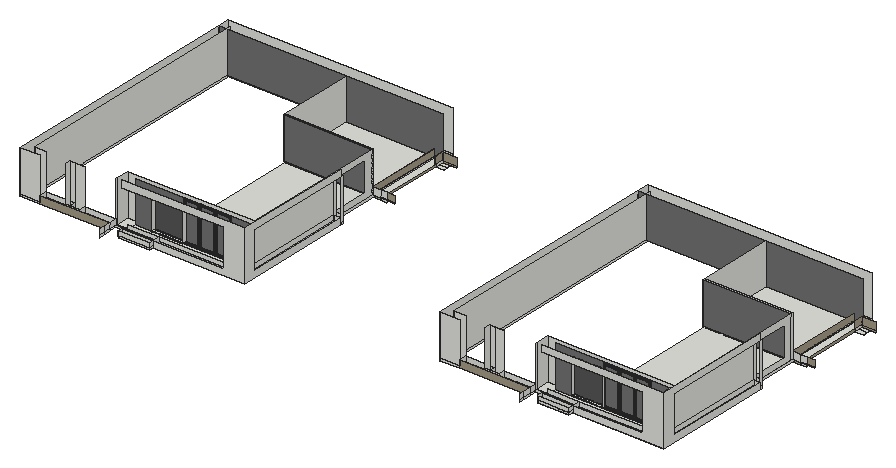
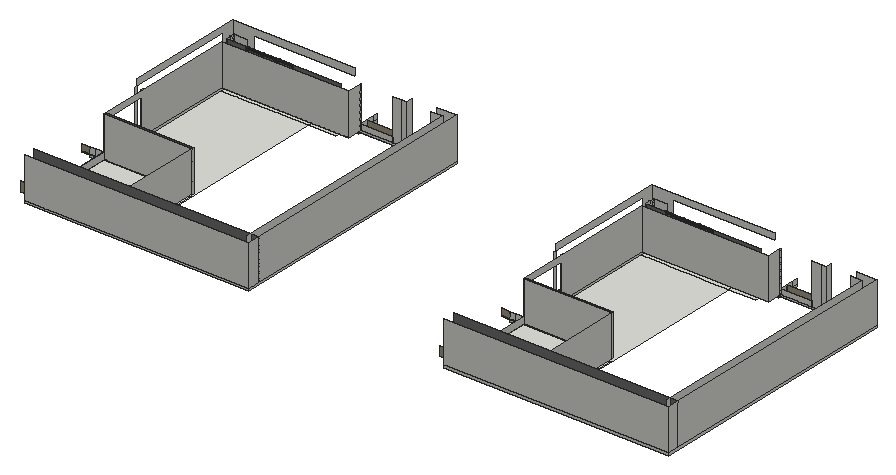
# SketchUp Ruby script. Lengths in inches.
U = 1.inch
M = Sketchup.active_model
def pt(a) = Geom::Point3d.new(a.map { |v| v * U })
def face(e, loops, mat)
  f = e.add_face(loops[0].map { |a| pt(a) })
  loops[1..].each { |l| e.add_face(l.map { |a| pt(a) }).erase! }
  f.material = f.back_material = mat if mat
  f
end
# faces: each face lists its corners as indices into pts; further lists are holes
def faces(e, pts, list, mat = nil) = list.each { |f| face(e, (f[0].is_a?(Array) ? f : [f]).map { |l| l.map { |i| pts[i] } }, mat) }
# xy, xz, yz: faces in a plane at the given z, y or x. An outline is a flat list of corners, or four numbers for a rectangle; further outlines are holes
def ring(l) = l.size == 4 ? [[l[0], l[1]], [l[2], l[1]], [l[2], l[3]], [l[0], l[3]]] : l.each_slice(2).to_a
def flat(e, list, mat, &to3) = list.each { |f| face(e, (f[0].is_a?(Array) ? f : [f]).map { |l| ring(l).map { |u, v| to3.(u, v) } }, mat) }
def xy(e, z, list, mat = nil) = flat(e, list, mat) { |x, y| [x, y, z] }
def xz(e, y, list, mat = nil) = flat(e, list, mat) { |x, z| [x, y, z] }
def yz(e, x, list, mat = nil) = flat(e, list, mat) { |y, z| [x, y, z] }
def lines(e, pts, list) = list.each { |a, b| e.add_line(pt(pts[a]), pt(pts[b])) }
# prism: a flat outline (further loops are holes) pulled along v
def prism(e, loops, v, mat = nil)
  f = face(e, loops, mat); d = Geom::Vector3d.new(v.map { |x| x * U })
  f.pushpull(f.normal.samedirection?(d) ? d.length : -d.length)
end
def box(e, o, s, mat = nil) = prism(e, [[o, [o[0] + s[0], o[1], o[2]], [o[0] + s[0], o[1] + s[1], o[2]], [o[0], o[1] + s[1], o[2]]]], [0, 0, s[2]], mat)
def at(x, y, z, deg = 0) = Geom::Transformation.translation(pt([x, y, z])) * Geom::Transformation.rotation(ORIGIN, Z_AXIS, deg.degrees)
def axes(o, x, y, z) = Geom::Transformation.new([*x, 0, *y, 0, *z, 0, *pt(o).to_a, 1])
def part(name) = M.definitions.add(name)
# library, detail: a bought-in or finely detailed component or shape, given as its bounding box
def library(name, o, s) = part(name).tap { |d| box(d.entities, o, s) }
def detail(e, o, s) = box(e.add_group.entities, o, s)
def put(e, d, t, mat = nil) = e.add_instance(d, t).tap { |i| i.material = mat if mat }
def group(e, t, mat = nil) = e.add_group.tap { |g| g.transformation = t; g.material = mat if mat }.entities
root = M.entities
M.materials.add("Wine2").color = [0, 0, 0]
M.materials["Wine2"].alpha = 0
M.materials.add("[0130_Gainsboro]").color = [39, 45, 50]
M.materials.add("[Color M05]").color = [114, 114, 114]
M.materials.add("[Color M06]").color = [86, 86, 86]
M.materials.add("[Concrete Tile]").color = [165, 155, 133]
M.materials.add("[Granite Brown]").color = [89, 59, 61]
c1 = part("Framed glazing panel")
xy(c1.entities,0,[[0,-0.98,43.07,0],[0,0,43.07,1.4]],"[0130_Gainsboro]")
xy(c1.entities,0.3,[[0.3,-1.43,42.77,-0.98]],"[0130_Gainsboro]")
xy(c1.entities,2.95,[[2.95,-1.43,40.12,-0.63],[2.95,-0.63,40.12,0],[2.95,0,40.12,0.64],[2.95,0.64,40.12,1.4]],"[0130_Gainsboro]")
xy(c1.entities,3.54,[[3.54,-0.63,39.53,0],[3.54,0,39.53,0.64]],"[0130_Gainsboro]")
xy(c1.entities,111.8125,[[3.54,-0.63,39.53,0],[3.54,0,39.53,0.64]],"[0130_Gainsboro]")
xy(c1.entities,112.4,[[2.95,-1.43,40.12,-0.63],[2.95,-0.63,40.12,0],[2.95,0,40.12,0.64],[2.95,0.64,40.12,1.4]],"[0130_Gainsboro]")
xy(c1.entities,115.05,[[0.3,-1.43,42.77,-0.98]],"[0130_Gainsboro]")
xy(c1.entities,115.35,[[0,-0.98,43.07,0],[0,0,43.07,1.4]],"[0130_Gainsboro]")
xz(c1.entities,-1.43,[[[0.3,0.3,42.77,115.05],[2.95,2.95,40.12,112.4]]],"[0130_Gainsboro]")
xz(c1.entities,-0.98,[[[0,0,43.07,115.35],[0.3,0.3,42.77,115.05]]],"[0130_Gainsboro]")
xz(c1.entities,-0.63,[[[2.95,2.95,40.12,112.4],[3.54,3.54,39.53,111.8125]]],"[0130_Gainsboro]")
xz(c1.entities,0,[[3.54,3.54,39.53,111.8125]],"Wine2")
xz(c1.entities,0,[[[0,0,43.07,115.35],[2.95,2.95,40.12,112.4]],[[2.95,2.95,40.12,112.4],[3.54,3.54,39.53,111.8125]]],"[0130_Gainsboro]")
xz(c1.entities,0.64,[[[2.95,2.95,40.12,112.4],[3.54,3.54,39.53,111.8125]]],"[0130_Gainsboro]")
xz(c1.entities,1.4,[[[0,0,43.07,115.35],[2.95,2.95,40.12,112.4]]],"[0130_Gainsboro]")
yz(c1.entities,0,[[-0.98,0,0,115.35],[0,0,1.4,115.35]],"[0130_Gainsboro]")
yz(c1.entities,0.3,[[-1.43,0.3,-0.98,115.05]],"[0130_Gainsboro]")
yz(c1.entities,2.95,[[-1.43,2.95,-0.63,112.4],[-0.63,2.95,0,112.4],[0,2.95,0.64,112.4],[0.64,2.95,1.4,112.4]],"[0130_Gainsboro]")
yz(c1.entities,3.54,[[-0.63,3.54,0,111.8125],[0,3.54,0.64,111.8125]],"[0130_Gainsboro]")
yz(c1.entities,39.53,[[-0.63,3.54,0,111.8125],[0,3.54,0.64,111.8125]],"[0130_Gainsboro]")
yz(c1.entities,40.12,[[-1.43,2.95,-0.63,112.4],[-0.63,2.95,0,112.4],[0,2.95,0.64,112.4],[0.64,2.95,1.4,112.4]],"[0130_Gainsboro]")
yz(c1.entities,42.77,[[-1.43,0.3,-0.98,115.05]],"[0130_Gainsboro]")
yz(c1.entities,43.07,[[-0.98,0,0,115.35],[0,0,1.4,115.35]],"[0130_Gainsboro]")
c2 = part("Glazed panel assembly")
put(c2.entities,c1,axes([90.57,1.43,0],[1.05148,0,0],[0,1,0],[0,0,1]))
put(c2.entities,c1,axes([0,1.43,0],[1.05148,0,0],[0,1,0],[0,0,1]))
put(c2.entities,c1,axes([45.29,1.43,0],[1.05148,0,0],[0,1,0],[0,0,1]))
xy(root,882,[[558.21,3201.66,648.68,3237.625],[1776.4,3201.66,1866.87,3237.625],[319.53,3214.625,319.53,3237.625,403.03,3237.625,403.03,3221.25,446.15,3221.25,446.15,3237.625,523.04,3237.625,523.04,3214.625],[648.68,3214.625,648.68,3237.625,890.875,3237.625,890.875,3257.1875,913.875,3257.1875,913.875,3214.625],[1537.72,3214.625,1537.72,3237.625,1621.22,3237.625,1621.22,3221.25,1664.33,3221.25,1664.33,3237.625,1741.23,3237.625,1741.23,3214.625],
  [1866.87,3214.625,1866.87,3237.625,2109.0625,3237.625,2109.0625,3257.1875,2132.0625,3257.1875,2132.0625,3214.625],[431.33,3221.25,446.15,3237.625],[1649.52,3221.25,1664.33,3237.625],[523.04,3237.625,557.4,3237.625,557.4,3241.3125,557.88,3241.3125,557.88,3244.9375,523.04,3244.9375],[648.68,3237.625,890.875,3237.625,890.875,3257.1875,635.3125,3257.1875,635.3125,3241.3125,648.68,3241.3125],
  [1741.23,3237.625,1775.59,3237.625,1775.59,3241.3125,1776.07,3241.3125,1776.07,3244.9375,1741.23,3244.9375],[1866.87,3237.625,2109.0625,3237.625,2109.0625,3257.1875,1853.5,3257.1875,1853.5,3241.3125,1866.87,3241.3125],[557.88,3241.3125,635.3125,3244.9375],[1776.07,3241.3125,1853.5,3244.9375],[557.88,3244.9375,635.3125,3257.1875],
  [1776.07,3244.9375,1853.5,3257.1875],[557.4,3257.1875,635.3125,3284.1875],[635.3125,3257.1875,890.875,3284.1875],[890.875,3257.1875,891.6875,3284.1875],[891.6875,3257.1875,894.3125,3563.51],
  [894.3125,3257.1875,913.875,3563.51],[1775.59,3257.1875,1853.5,3284.1875],[1853.5,3257.1875,2109.0625,3284.1875],[2109.0625,3257.1875,2109.875,3284.1875],[2109.875,3257.1875,2112.5,3563.51],
  [2112.5,3257.1875,2132.0625,3563.51],[635.3125,3284.1875,890.875,3710.5625],[1853.5,3284.1875,2109.0625,3710.5625],[894,3563.51,894.3125,3570.7],[894.3125,3563.51,913.875,3570.7],
  [2112.1875,3563.51,2112.5,3570.7],[2112.5,3563.51,2132.0625,3570.7],[635.3125,3710.5625,637.0625,3933.57],[637.0625,3710.5625,637.0625,3933.57,889.625,3933.57,889.625,3907.5625,890.875,3907.5625,890.875,3710.5625],[1853.5,3710.5625,1855.25,3933.57],
  [1855.25,3710.5625,1855.25,3933.57,2107.8125,3933.57,2107.8125,3907.5625,2109.0625,3907.5625,2109.0625,3710.5625],[889.625,3907.5625,890.875,3933.57],[890.875,3907.5625,912.625,3920.25],[912.625,3907.5625,913.875,3920.25],[913.875,3907.5625,938.375,3920.25],
  [938.375,3907.5625,938.5625,3933.57],[2107.8125,3907.5625,2109.0625,3933.57],[2109.0625,3907.5625,2130.8125,3920.25],[2130.8125,3907.5625,2132.0625,3920.25],[2132.0625,3907.5625,2156.5625,3920.25],
  [2156.5625,3907.5625,2156.75,3933.57],[890.875,3920.25,912.625,3933.57],[912.625,3920.25,913.875,3933.57],[913.875,3920.25,938.375,3933.57],[2109.0625,3920.25,2130.8125,3933.57],
  [2130.8125,3920.25,2132.0625,3933.57],[2132.0625,3920.25,2156.5625,3933.57],[635.3125,3933.57,890.875,3946.0625],[1853.5,3933.57,2109.0625,3946.0625]])
xy(root,882,[[890.875,3710.5625,913.875,3907.5625],[2109.0625,3710.5625,2132.0625,3907.5625]],"[Concrete Tile]")
xy(root,882,[[557.4,3237.625,557.88,3241.3125],[1775.59,3237.625,1776.07,3241.3125]],"[Granite Brown]")
xy(root,888,[[557.88,3201.66,558.21,3214.625],[558.21,3201.66,647.87,3214.625],[647.87,3201.66,648.68,3214.625],[1776.07,3201.66,1776.4,3214.625],[1776.4,3201.66,1866.06,3214.625],
  [1866.06,3201.66,1866.87,3214.625],[557.88,3214.625,558.21,3237.625],[558.21,3214.625,647.87,3237.625],[647.87,3214.625,648.68,3237.625],[1776.07,3214.625,1776.4,3237.625],
  [1776.4,3214.625,1866.06,3237.625],[1866.06,3214.625,1866.87,3237.625],[523.04,3237.625,557.4,3241.3125],[648.68,3237.625,890.875,3241.3125],[1741.23,3237.625,1775.59,3241.3125],
  [1866.87,3237.625,2109.0625,3241.3125],[523.04,3241.3125,523.04,3280.4375,557.4,3280.4375,557.4,3265.625,557.88,3265.625,557.88,3241.3125],[557.88,3241.3125,890.875,3265.625],[1741.23,3241.3125,1741.23,3280.4375,1775.59,3280.4375,1775.59,3265.625,1776.07,3265.625,1776.07,3241.3125],[1776.07,3241.3125,2109.0625,3265.625],
  [557.4,3265.625,890.875,3280.4375],[1775.59,3265.625,2109.0625,3280.4375],[894.3125,3563.51,913.875,3570.7],[2112.5,3563.51,2132.0625,3570.7],[635.3125,3704.6875,890.875,3710.5625],
  [1853.5,3704.6875,2109.0625,3710.5625],[890.875,3710.5625,890.875,3931.82,912.625,3931.82,912.625,3907.5625,913.875,3907.5625,913.875,3710.5625],[2109.0625,3710.5625,2109.0625,3931.82,2130.8125,3931.82,2130.8125,3907.5625,2132.0625,3907.5625,2132.0625,3710.5625],[912.625,3907.5625,913.875,3931.82],[2130.8125,3907.5625,2132.0625,3931.82],
  [890.875,3931.82,912.625,3933.32],[912.625,3931.82,913.875,3933.32],[2109.0625,3931.82,2130.8125,3933.32],[2130.8125,3931.82,2132.0625,3933.32],[890.875,3933.32,912.625,3933.57],
  [912.625,3933.32,913.875,3933.57],[2109.0625,3933.32,2130.8125,3933.57],[2130.8125,3933.32,2132.0625,3933.57],[285.875,3933.8125,890.875,3946.0625],[1504.0625,3933.8125,2109.0625,3946.0625]])
xy(root,888,[[557.4,3201.66,557.88,3214.625],[1775.59,3201.66,1776.07,3214.625],[557.4,3237.625,557.88,3241.3125],[1775.59,3237.625,1776.07,3241.3125]],"[Granite Brown]")
xy(root,889.75,[[635.3125,3710.5625,889.625,3931.82],[889.625,3710.5625,890.875,3931.82],[1853.5,3710.5625,2107.8125,3931.82],[2107.8125,3710.5625,2109.0625,3931.82]])
xy(root,895.375,[[632.49,3257.1875,648.79,3265.625],[648.79,3257.1875,650.48,3265.625],[650.48,3257.1875,701.59,3265.625],[1850.67,3257.1875,1866.98,3265.625],[1866.98,3257.1875,1868.66,3265.625],
  [1868.66,3257.1875,1919.77,3265.625]])
xy(root,895.6875,[[611.65,3257.1875,632.49,3265.625],[1829.84,3257.1875,1850.67,3265.625]])
xz(root,3201.66,[[558.21,882,648.68,888],[1776.4,882,1866.87,888],[557.88,888,647.87,900.6875],[1776.07,888,1866.06,900.6875]])
xz(root,3201.66,[[557.4,888,557.88,900.6875],[1775.59,888,1776.07,900.6875]],"[Granite Brown]")
xz(root,3214.625,[[262.875,882,319.53,888],[648.68,882,913.875,882,913.875,1026.6875,557.88,1026.6875,557.88,1008,852.99,1008,852.99,900.6875,647.87,900.6875,647.87,888,648.68,888],[1481.0625,882,1537.72,888],[1866.87,882,2132.0625,882,2132.0625,1026.6875,1776.07,1026.6875,1776.07,1008,2071.18,1008,2071.18,900.6875,1866.06,900.6875,1866.06,888,1866.87,888],[262.875,888,319.53,1008],
  [557.4,888,647.87,900.6875],[1481.0625,888,1537.72,1008],[1775.59,888,1866.06,900.6875]])
xz(root,3214.625,[[319.53,882,523.04,903.4375],[1537.72,882,1741.23,903.4375]],"[Concrete Tile]")
xz(root,3221.25,[[403.0625,888,403.0625,903.4375,388.33,903.51,388.25,888.07],[403.0625,888,403.14,903.4375,403.0625,903.4375],[403.0625,888,431.33,888,431.33,903.4375,403.14,903.4375],[1621.25,888,1621.25,903.4375,1606.52,903.51,1606.4375,888.07],[1621.25,888,1621.33,903.4375,1621.25,903.4375],
  [1621.25,888,1649.52,888,1649.52,903.4375,1621.33,903.4375]])
xz(root,3237.625,[[285.875,882,557.4,888],[558.21,882,648.68,888],[648.68,882,890.875,888],[1504.0625,882,1775.59,888],[1776.4,882,1866.87,888],
  [1866.87,882,2109.0625,888],[285.875,888,319.53,1008],[319.53,888,403.0625,888,388.25,888.07,388.33,903.4375,319.53,903.4375],[403.0625,888,388.25,888.07,388.33,903.4375,403.0625,903.4375],[403.0625,888,403.66,1008,388.85,1008,388.33,903.4375,403.0625,903.4375],
  [403.0625,888,403.66,1008,431.33,1008,431.33,888],[431.33,888,523.04,903.4375],[557.88,888,647.87,900.6875],[647.87,888,647.87,900.6875,852.99,900.6875,852.99,1008,890.875,1008,890.875,888],[1504.0625,888,1537.72,1008],
  [1537.72,888,1621.25,888,1606.4375,888.07,1606.52,903.4375,1537.72,903.4375],[1621.25,888,1606.4375,888.07,1606.52,903.4375,1621.25,903.4375],[1621.25,888,1621.85,1008,1607.04,1008,1606.52,903.4375,1621.25,903.4375],[1621.25,888,1621.85,1008,1649.52,1008,1649.52,888],[1649.52,888,1741.23,903.4375],
  [1776.07,888,1866.06,900.6875],[1866.06,888,1866.06,900.6875,2071.18,900.6875,2071.18,1008,2109.0625,1008,2109.0625,888]])
xz(root,3237.625,[[557.4,882,557.88,888],[1775.59,882,1776.07,888]],"[Granite Brown]")
xz(root,3241.3125,[[557.4,882,648.68,888],[1775.59,882,1866.87,888]])
xz(root,3249.875,[[890.875,888,894.3125,1008],[2109.0625,888,2112.5,1008]])
xz(root,3257.1875,[[632.49,893.4375,701.59,893.4375,701.59,895.375,632.49,895.375,632.49,895.6875,611.65,895.6875,611.65,893.75,632.49,893.75],[1850.67,893.4375,1919.77,893.4375,1919.77,895.375,1850.67,895.375,1850.67,895.6875,1829.84,895.6875,1829.84,893.75,1850.67,893.75]])
xz(root,3265.625,[[[557.88,888,890.875,888,890.875,1008,557.88,1008,557.88,986.96,557.4,986.96,557.4,934.68,557.88,934.68],[632.49,895.375,632.49,895.6875,611.65,895.6875,611.65,991.5625,701.59,991.5625,701.59,895.375]],[[1776.07,888,2109.0625,888,2109.0625,1008,1776.07,1008,1776.07,986.96,1775.59,986.96,1775.59,934.68,1776.07,934.68],[1850.67,895.375,1850.67,895.6875,1829.84,895.6875,1829.84,991.5625,1919.77,991.5625,1919.77,895.375]]],"[Color M05]")
xz(root,3265.625,[[632.49,895.375,701.59,895.375,701.59,991.5625,611.65,991.5625,611.65,895.6875,632.49,895.6875],[1850.67,895.375,1919.77,895.375,1919.77,991.5625,1829.84,991.5625,1829.84,895.6875,1850.67,895.6875]],"[Color M06]")
xz(root,3280.4375,[[523.04,888,890.875,1008],[1741.23,888,2109.0625,1008]])
xz(root,3563.51,[[894.3125,882,913.875,888],[2112.5,882,2132.0625,888],[894.3125,888,913.875,900.6875],[2112.5,888,2132.0625,900.6875]])
xz(root,3570.7,[[894.3125,882,913.875,888],[2112.5,882,2132.0625,888],[894.3125,888,913.875,905.36],[2112.5,888,2132.0625,905.36]])
xz(root,3704.6875,[[635.3125,888,890.875,1008],[1853.5,888,2109.0625,1008]],"[Color M05]")
xz(root,3710.5625,[[913.875,882,930.75,888],[2132.0625,882,2148.9375,888],[635.3125,888,890.875,889.75],[890.875,888,913.875,908.8125],[913.875,888,930.75,889.75],
  [930.75,888,954.6875,889.75],[1853.5,888,2109.0625,889.75],[2109.0625,888,2132.0625,908.8125],[2132.0625,888,2148.9375,889.75],[2148.9375,888,2172.875,889.75],
  [635.3125,889.75,635.3125,1008,890.875,1008,890.875,908.8125,889.625,908.8125,889.625,889.75],[889.625,889.75,890.875,908.8125],[913.875,889.75,930.75,908.8125],[1853.5,889.75,1853.5,1008,2109.0625,1008,2109.0625,908.8125,2107.8125,908.8125,2107.8125,889.75],[2107.8125,889.75,2109.0625,908.8125],
  [2132.0625,889.75,2148.9375,908.8125]])
xz(root,3710.5625,[[930.75,889.75,954.6875,908.8125],[2148.9375,889.75,2172.875,908.8125]],"[Concrete Tile]")
xz(root,3907.5625,[[912.625,882,913.875,888],[2130.8125,882,2132.0625,888],[912.625,888,913.875,908.8125],[2130.8125,888,2132.0625,908.8125]])
xz(root,3931.82,[[889.625,889.75,890.875,908.8125],[2107.8125,889.75,2109.0625,908.8125]])
xz(root,3933.32,[[912.625,888,913.875,908.8125],[2130.8125,888,2132.0625,908.8125]])
xz(root,3933.57,[[912.625,882,913.875,888],[2130.8125,882,2132.0625,888]])
xz(root,3933.57,[[913.875,882,954.6875,908.8125],[2132.0625,882,2172.875,908.8125]],"[Concrete Tile]")
xz(root,3933.8125,[[262.875,888,913.875,1008],[1481.0625,888,2132.0625,1008]],"[Color M05]")
xz(root,3946.0625,[[285.875,882,890.875,888],[1504.0625,882,2109.0625,888]])
xz(root,3969.0625,[[262.875,882,913.875,888],[1481.0625,882,2132.0625,888],[262.875,888,913.875,1008],[1481.0625,888,2132.0625,1008]])
yz(root,262.875,[[3214.625,882,3969.0625,888],[3214.625,888,3933.8125,1008],[3933.8125,888,3969.0625,1008]])
yz(root,285.875,[[3237.625,882,3946.0625,888],[3237.625,888,3946.0625,1008]])
yz(root,319.53,[[3214.625,888,3237.625,903.4375]])
yz(root,403.0625,[[3221.25,888,3237.625,903.4375]])
yz(root,431.33,[[3221.25,888,3237.625,903.4375]])
yz(root,523.04,[[3177.9375,882,3214.625,888],[3177.9375,888,3214.625,903.4375],[3214.625,888,3237.625,903.4375],[3237.625,888,3241.3125,1008],[3241.3125,888,3280.4375,1008]])
yz(root,557.4,[[3237.625,882,3241.3125,888],[3201.66,888,3214.625,900.6875]])
yz(root,558.21,[[3201.66,882,3237.625,888]])
yz(root,611.65,[[3257.1875,895.6875,3265.625,991.5625]])
yz(root,632.49,[[3257.1875,895.375,3265.625,895.6875]])
yz(root,635.3125,[[3704.6875,888,3710.5625,1008],[3710.5625,889.75,3931.82,1008]])
yz(root,647.87,[[3201.66,888,3214.625,900.6875],[3214.625,888,3237.625,900.6875]])
yz(root,648.68,[[3201.66,882,3214.625,888],[3214.625,882,3237.625,888],[3237.625,882,3241.3125,888]])
yz(root,701.59,[[3257.1875,895.375,3265.625,991.5625]])
yz(root,889.625,[[3710.5625,889.75,3931.82,908.8125]])
yz(root,890.875,[[3237.625,882,3946.0625,888],[3237.625,888,3241.3125,1008],[3241.3125,888,3249.875,1008],[3249.875,888,3265.625,1008],[[3280.4375,888,3704.6875,1008],[3570.7,905.36,3681.01,991.04]],
  [3704.6875,888,3710.5625,889.75],[3710.5625,888,3931.82,889.75],[3931.82,888,3933.32,889.75],[3933.32,888,3933.57,889.75],[3704.6875,889.75,3710.5625,1008]])
yz(root,890.875,[[3710.5625,889.75,3931.82,908.8125]],"[Concrete Tile]")
yz(root,894.3125,[[3563.51,882,3570.7,888],[3249.875,888,3563.51,900.6875],[3563.51,888,3570.7,1008]])
yz(root,912.625,[[3907.5625,882,3933.57,888],[3907.5625,888,3933.32,908.8125]])
yz(root,913.875,[[3214.625,882,3563.51,882,3563.51,900.6875,3249.875,900.6875,3249.875,1008,3563.51,1008,3563.51,1026.6875,3214.625,1026.6875],[3563.51,882,3570.7,888],[3907.5625,882,3933.57,888],[3933.57,882,3934.82,888],[3563.51,888,3570.7,1008],
  [3933.32,888,3933.57,908.8125],[3933.57,888,3933.8125,908.8125],[3933.8125,888,3934.82,908.8125]])
yz(root,913.875,[[3710.5625,882,3907.5625,888],[3907.5625,888,3933.32,908.8125]],"[Concrete Tile]")
yz(root,1481.0625,[[3214.625,882,3969.0625,888],[3214.625,888,3933.8125,1008],[3933.8125,888,3969.0625,1008]])
yz(root,1504.0625,[[3237.625,882,3946.0625,888],[3237.625,888,3946.0625,1008]])
yz(root,1537.72,[[3214.625,888,3237.625,903.4375]])
yz(root,1621.25,[[3221.25,888,3237.625,903.4375]])
yz(root,1649.52,[[3221.25,888,3237.625,903.4375]])
yz(root,1741.23,[[3177.9375,882,3214.625,888],[3177.9375,888,3214.625,903.4375],[3214.625,888,3237.625,903.4375],[3237.625,888,3241.3125,1008],[3241.3125,888,3280.4375,1008]])
yz(root,1775.59,[[3237.625,882,3241.3125,888],[3201.66,888,3214.625,900.6875]])
yz(root,1776.4,[[3201.66,882,3237.625,888]])
yz(root,1829.84,[[3257.1875,895.6875,3265.625,991.5625]])
yz(root,1850.67,[[3257.1875,895.375,3265.625,895.6875]])
yz(root,1853.5,[[3704.6875,888,3710.5625,1008],[3710.5625,889.75,3931.82,1008]])
yz(root,1866.06,[[3201.66,888,3214.625,900.6875],[3214.625,888,3237.625,900.6875]])
yz(root,1866.87,[[3201.66,882,3214.625,888],[3214.625,882,3237.625,888],[3237.625,882,3241.3125,888]])
yz(root,1919.77,[[3257.1875,895.375,3265.625,991.5625]])
yz(root,2107.8125,[[3710.5625,889.75,3931.82,908.8125]])
yz(root,2109.0625,[[3237.625,882,3946.0625,888],[3237.625,888,3241.3125,1008],[3241.3125,888,3249.875,1008],[3249.875,888,3265.625,1008],[[3280.4375,888,3704.6875,1008],[3570.7,905.36,3681.01,991.04]],
  [3704.6875,888,3710.5625,889.75],[3710.5625,888,3931.82,889.75],[3931.82,888,3933.32,889.75],[3933.32,888,3933.57,889.75],[3704.6875,889.75,3710.5625,1008]])
yz(root,2109.0625,[[3710.5625,889.75,3931.82,908.8125]],"[Concrete Tile]")
yz(root,2112.5,[[3563.51,882,3570.7,888],[3249.875,888,3563.51,900.6875],[3563.51,888,3570.7,1008]])
yz(root,2130.8125,[[3907.5625,882,3933.57,888],[3907.5625,888,3933.32,908.8125]])
yz(root,2132.0625,[[3214.625,882,3563.51,882,3563.51,900.6875,3249.875,900.6875,3249.875,1008,3563.51,1008,3563.51,1026.6875,3214.625,1026.6875],[3563.51,882,3570.7,888],[3907.5625,882,3933.57,888],[3933.57,882,3934.82,888],[3563.51,888,3570.7,1008],
  [3933.32,888,3933.57,908.8125],[3933.57,888,3933.8125,908.8125],[3933.8125,888,3934.82,908.8125]])
yz(root,2132.0625,[[3710.5625,882,3907.5625,888],[3907.5625,888,3933.32,908.8125]],"[Concrete Tile]")
p = [[403.0625,3237.625,888],[403.0625,3221.25,888],[388.25,3221.25,888.07],[388.25,3237.625,888.07],[1621.25,3237.625,888],[1621.25,3221.25,888],
  [1606.4375,3221.25,888.07],[1606.4375,3237.625,888.07],[388.33,3221.25,903.51],[388.85,3221.25,1008.07],[388.85,3237.625,1008.07],[388.85,3237.625,1008],
  [388.33,3237.625,903.4375],[1606.52,3221.25,903.51],[1607.04,3221.25,1008.07],[1607.04,3237.625,1008.07],[1607.04,3237.625,1008],[1606.52,3237.625,903.4375],
  [1741.23,3193,888],[1741.23,3193,903.4375],[1741.23,3193,882],[2132.0625,3931.82,888],[2172.875,3931.82,888],[913.875,3931.82,888],
  [954.6875,3931.82,888],[523.04,3193,882],[523.04,3193,888],[523.04,3193,903.4375]]
faces(root,p,[[0,1,2,3],[4,5,6,7],[3,2,8,9,10,11,12],[7,6,13,14,15,16,17]])
lines(root,p,[[18,19],[20,18],[21,22],[23,24],[25,26],[26,27]])
put(root,c2,at(1916.05,3263.55,891.83))
put(root,c2,at(697.86,3263.55,891.83))
